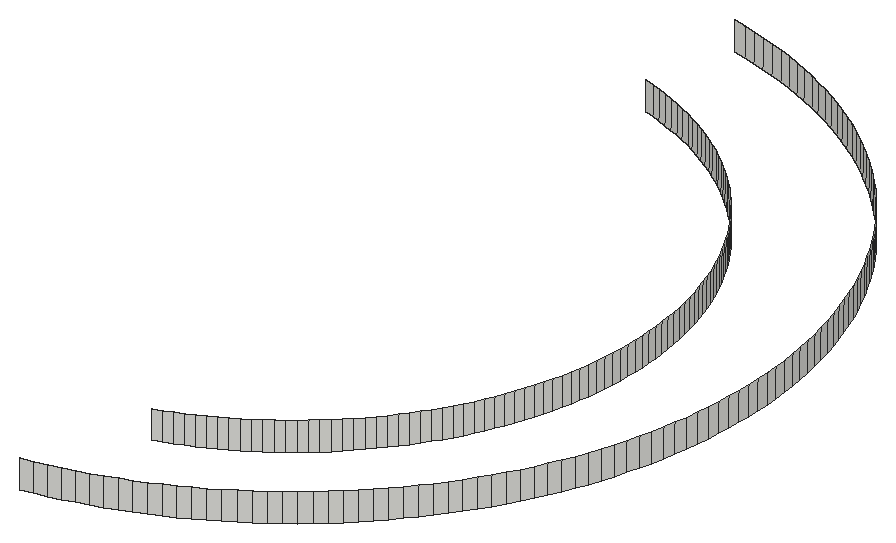
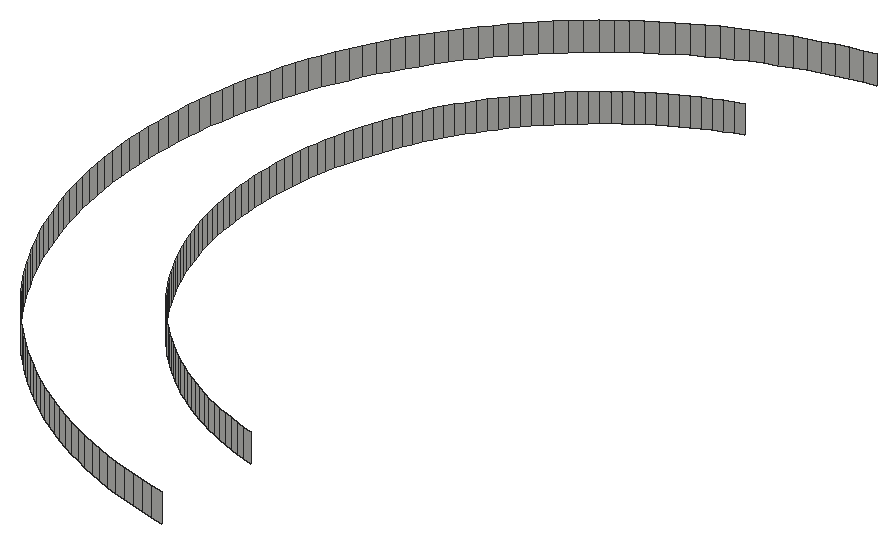
# SketchUp Ruby script. Lengths in inches.
U = 1.inch
M = Sketchup.active_model
def pt(a) = Geom::Point3d.new(a.map { |v| v * U })
def face(e, loops, mat)
  f = e.add_face(loops[0].map { |a| pt(a) })
  loops[1..].each { |l| e.add_face(l.map { |a| pt(a) }).erase! }
  f.material = f.back_material = mat if mat
  f
end
# faces: each face lists its corners as indices into pts; further lists are holes
def faces(e, pts, list, mat = nil) = list.each { |f| face(e, (f[0].is_a?(Array) ? f : [f]).map { |l| l.map { |i| pts[i] } }, mat) }
# xy, xz, yz: faces in a plane at the given z, y or x. An outline is a flat list of corners, or four numbers for a rectangle; further outlines are holes
def ring(l) = l.size == 4 ? [[l[0], l[1]], [l[2], l[1]], [l[2], l[3]], [l[0], l[3]]] : l.each_slice(2).to_a
def flat(e, list, mat, &to3) = list.each { |f| face(e, (f[0].is_a?(Array) ? f : [f]).map { |l| ring(l).map { |u, v| to3.(u, v) } }, mat) }
def xy(e, z, list, mat = nil) = flat(e, list, mat) { |x, y| [x, y, z] }
def xz(e, y, list, mat = nil) = flat(e, list, mat) { |x, z| [x, y, z] }
def yz(e, x, list, mat = nil) = flat(e, list, mat) { |y, z| [x, y, z] }
def lines(e, pts, list) = list.each { |a, b| e.add_line(pt(pts[a]), pt(pts[b])) }
# prism: a flat outline (further loops are holes) pulled along v
def prism(e, loops, v, mat = nil)
  f = face(e, loops, mat); d = Geom::Vector3d.new(v.map { |x| x * U })
  f.pushpull(f.normal.samedirection?(d) ? d.length : -d.length)
end
def box(e, o, s, mat = nil) = prism(e, [[o, [o[0] + s[0], o[1], o[2]], [o[0] + s[0], o[1] + s[1], o[2]], [o[0], o[1] + s[1], o[2]]]], [0, 0, s[2]], mat)
def at(x, y, z, deg = 0) = Geom::Transformation.translation(pt([x, y, z])) * Geom::Transformation.rotation(ORIGIN, Z_AXIS, deg.degrees)
def axes(o, x, y, z) = Geom::Transformation.new([*x, 0, *y, 0, *z, 0, *pt(o).to_a, 1])
def part(name) = M.definitions.add(name)
# library, detail: a bought-in or finely detailed component or shape, given as its bounding box
def library(name, o, s) = part(name).tap { |d| box(d.entities, o, s) }
def detail(e, o, s) = box(e.add_group.entities, o, s)
def put(e, d, t, mat = nil) = e.add_instance(d, t).tap { |i| i.material = mat if mat }
def group(e, t, mat = nil) = e.add_group.tap { |g| g.transformation = t; g.material = mat if mat }.entities
root = M.entities
p = [[923.47,230.86,117.3125],[925.9375,231.35,117.3125],[925.9375,231.35,111.3125],[923.47,230.86,111.3125],[928.39,231.91,117.3125],[928.39,231.91,111.3125],
  [930.83,232.53,117.3125],[930.83,232.53,111.3125],[933.24,233.21,117.3125],[933.24,233.21,111.3125],[935.64,233.95,117.3125],[935.64,233.95,111.3125],
  [938.02,234.76,117.3125],[938.02,234.76,111.3125],[940.38,235.63,117.3125],[940.38,235.63,111.3125],[942.72,236.5625,117.3125],[942.72,236.5625,111.3125],
  [945.03,237.56,117.3125],[945.03,237.56,111.3125],[947.31,238.61,117.3125],[947.31,238.61,111.3125],[949.5625,239.72,117.3125],[949.5625,239.72,111.3125],
  [951.79,240.89,117.3125],[951.79,240.89,111.3125],[953.98,242.12,117.3125],[953.98,242.12,111.3125],[956.14,243.4,117.3125],[956.14,243.4,111.3125],
  [958.26,244.74,117.3125],[958.26,244.74,111.3125],[960.35,246.14,117.3125],[960.35,246.14,111.3125],[962.41,247.59,117.3125],[962.41,247.59,111.3125],
  [964.42,249.09,117.3125],[964.42,249.09,111.3125],[966.39,250.65,117.3125],[966.39,250.65,111.3125],[968.33,252.26,117.3125],[968.33,252.26,111.3125],
  [970.22,253.91,117.3125],[970.22,253.91,111.3125],[972.0625,255.62,117.3125],[972.0625,255.62,111.3125],[973.86,257.375,117.3125],[973.86,257.375,111.3125],
  [931.78,258.04,117.3125],[930.01,257.39,117.3125],[930.01,257.39,111.3125],[931.78,258.04,111.3125],[975.61,259.17,117.3125],[975.61,259.17,111.3125],
  [933.53,258.74,117.3125],[933.53,258.74,111.3125],[935.26,259.48,117.3125],[935.26,259.48,111.3125],[977.32,261.02,117.3125],[977.32,261.02,111.3125],
  [936.98,260.27,117.3125],[936.98,260.27,111.3125],[938.67,261.1,117.3125],[938.67,261.1,111.3125],[978.98,262.91,117.3125],[978.98,262.91,111.3125],
  [940.33,261.98,117.3125],[940.33,261.98,111.3125],[941.98,262.9,117.3125],[941.98,262.9,111.3125],[943.6,263.87,117.3125],[943.6,263.87,111.3125],
  [980.58,264.84,117.3125],[980.58,264.84,111.3125],[945.19,264.87,117.3125],[945.19,264.87,111.3125],[982.14,266.82,117.3125],[982.14,266.82,111.3125],
  [946.76,265.92,117.3125],[946.76,265.92,111.3125],[948.3,267.01,117.3125],[948.3,267.01,111.3125],[983.64,268.83,117.3125],[983.64,268.83,111.3125],
  [949.81,268.13,117.3125],[949.81,268.13,111.3125],[951.29,269.3,117.3125],[951.29,269.3,111.3125],[985.09,270.88,117.3125],[985.09,270.88,111.3125],
  [952.74,270.51,117.3125],[952.74,270.51,111.3125],[954.16,271.75,117.3125],[954.16,271.75,111.3125],[986.49,272.97,117.3125],[986.49,272.97,111.3125],
  [955.54,273.03,117.3125],[955.54,273.03,111.3125],[956.89,274.34,117.3125],[956.89,274.34,111.3125],[987.83,275.1,117.3125],[987.83,275.1,111.3125],
  [958.21,275.69,117.3125],[958.21,275.69,111.3125],[989.12,277.26,117.3125],[989.12,277.26,111.3125],[959.49,277.08,117.3125],[959.49,277.08,111.3125],
  [960.73,278.5,117.3125],[960.73,278.5,111.3125],[990.35,279.45,117.3125],[990.35,279.45,111.3125],[961.93,279.95,117.3125],[961.93,279.95,111.3125],
  [991.52,281.67,117.3125],[991.52,281.67,111.3125],[963.1,281.43,117.3125],[963.1,281.43,111.3125],[964.23,282.9375,117.3125],[964.23,282.9375,111.3125],
  [992.625,283.93,117.3125],[992.625,283.93,111.3125],[965.32,284.47,117.3125],[965.32,284.47,111.3125],[993.68,286.21,117.3125],[993.68,286.21,111.3125],
  [966.36,286.04,117.3125],[966.36,286.04,111.3125],[967.37,287.64,117.3125],[967.37,287.64,111.3125],[994.67,288.52,117.3125],[994.67,288.52,111.3125],
  [968.33,289.26,117.3125],[968.33,289.26,111.3125],[995.6,290.85,117.3125],[995.6,290.85,111.3125],[969.25,290.9,117.3125],[969.25,290.9,111.3125],
  [970.13,292.57,117.3125],[970.13,292.57,111.3125],[996.47,293.21,117.3125],[996.47,293.21,111.3125],[970.96,294.26,117.3125],[970.96,294.26,111.3125],
  [997.28,295.59,117.3125],[997.28,295.59,111.3125],[971.75,295.97,117.3125],[971.75,295.97,111.3125],[998.03,297.99,117.3125],[998.03,297.99,111.3125],
  [972.5,297.7,117.3125],[972.5,297.7,111.3125],[973.2,299.45,117.3125],[973.2,299.45,111.3125],[998.71,300.41,117.3125],[998.71,300.41,111.3125],
  [973.85,301.22,117.3125],[973.85,301.22,111.3125],[999.33,302.85,117.3125],[999.33,302.85,111.3125],[974.45,303.01,117.3125],[974.45,303.01,111.3125],
  [999.88,305.3,117.3125],[999.88,305.3,111.3125],[975.01,304.81,117.3125],[975.01,304.81,111.3125],[975.53,306.62,117.3125],[975.53,306.62,111.3125],
  [1000.37,307.76,117.3125],[1000.37,307.76,111.3125],[975.99,308.45,117.3125],[975.99,308.45,111.3125],[1000.8,310.24,117.3125],[1000.8,310.24,111.3125],
  [976.41,310.29,117.3125],[976.41,310.29,111.3125],[1001.16,312.73,117.3125],[1001.16,312.73,111.3125],[976.77,312.14,117.3125],[976.77,312.14,111.3125],
  [977.09,313.99,117.3125],[977.09,313.99,111.3125],[1001.45,315.22,117.3125],[1001.45,315.22,111.3125],[977.36,315.86,117.3125],[977.36,315.86,111.3125],
  [1001.68,317.72,117.3125],[1001.68,317.72,111.3125],[977.58,317.73,117.3125],[977.58,317.73,111.3125],[977.76,319.61,117.3125],[977.76,319.61,111.3125],
  [1001.85,320.23,117.3125],[1001.85,320.23,111.3125],[977.88,321.49,117.3125],[977.88,321.49,111.3125],[1001.95,322.74,117.3125],[1001.95,322.74,111.3125],
  [977.95,323.37,117.3125],[977.95,323.37,111.3125],[1001.98,325.26,117.3125],[1001.98,325.26,111.3125],[977.98,325.26,117.3125],[977.98,325.26,111.3125],
  [977.95,327.14,117.3125],[977.95,327.14,111.3125],[1001.95,327.77,117.3125],[1001.95,327.77,111.3125],[977.88,329.02,117.3125],[977.88,329.02,111.3125],
  [1001.85,330.28,117.3125],[1001.85,330.28,111.3125],[977.76,330.91,117.3125],[977.76,330.91,111.3125],[1001.68,332.79,117.3125],[1001.68,332.79,111.3125],
  [977.58,332.78,117.3125],[977.58,332.78,111.3125],[977.36,334.65,117.3125],[977.36,334.65,111.3125],[1001.45,335.29,117.3125],[1001.45,335.29,111.3125],
  [977.09,336.52,117.3125],[977.09,336.52,111.3125],[1001.16,337.79,117.3125],[1001.16,337.79,111.3125],[976.77,338.38,117.3125],[976.77,338.38,111.3125],
  [1000.8,340.27,117.3125],[1000.8,340.27,111.3125],[976.41,340.23,117.3125],[976.41,340.23,111.3125],[975.99,342.0625,117.3125],[975.99,342.0625,111.3125],
  [1000.37,342.75,117.3125],[1000.37,342.75,111.3125],[975.53,343.89,117.3125],[975.53,343.89,111.3125],[999.88,345.22,117.3125],[999.88,345.22,111.3125],
  [975.01,345.71,117.3125],[975.01,345.71,111.3125],[999.33,347.67,117.3125],[999.33,347.67,111.3125],[974.45,347.51,117.3125],[974.45,347.51,111.3125],
  [973.85,349.29,117.3125],[973.85,349.29,111.3125],[998.71,350.1,117.3125],[998.71,350.1,111.3125],[973.2,351.06,117.3125],[973.2,351.06,111.3125],
  [998.03,352.52,117.3125],[998.03,352.52,111.3125],[972.5,352.81,117.3125],[972.5,352.81,111.3125],[997.28,354.92,117.3125],[997.28,354.92,111.3125],
  [971.75,354.54,117.3125],[971.75,354.54,111.3125],[970.96,356.25,117.3125],[970.96,356.25,111.3125],[996.47,357.3,117.3125],[996.47,357.3,111.3125],
  [970.13,357.94,117.3125],[970.13,357.94,111.3125],[995.6,359.66,117.3125],[995.6,359.66,111.3125],[969.25,359.61,117.3125],[969.25,359.61,111.3125],
  [968.33,361.26,117.3125],[968.33,361.26,111.3125],[994.67,361.99,117.3125],[994.67,361.99,111.3125],[967.37,362.875,117.3125],[967.37,362.875,111.3125],
  [993.68,364.3,117.3125],[993.68,364.3,111.3125],[966.36,364.47,117.3125],[966.36,364.47,111.3125],[992.625,366.59,117.3125],[992.625,366.59,111.3125],
  [965.32,366.04,117.3125],[965.32,366.04,111.3125],[964.23,367.58,117.3125],[964.23,367.58,111.3125],[991.52,368.84,117.3125],[991.52,368.84,111.3125],
  [963.1,369.09,117.3125],[963.1,369.09,111.3125],[990.35,371.0625,117.3125],[990.35,371.0625,111.3125],[961.93,370.57,117.3125],[961.93,370.57,111.3125],
  [960.73,372.02,117.3125],[960.73,372.02,111.3125],[989.12,373.26,117.3125],[989.12,373.26,111.3125],[959.49,373.43,117.3125],[959.49,373.43,111.3125],
  [987.83,375.42,117.3125],[987.83,375.42,111.3125],[958.21,374.82,117.3125],[958.21,374.82,111.3125],[956.89,376.17,117.3125],[956.89,376.17,111.3125],
  [986.49,377.54,117.3125],[986.49,377.54,111.3125],[955.54,377.48,117.3125],[955.54,377.48,111.3125],[954.16,378.76,117.3125],[954.16,378.76,111.3125],
  [985.09,379.63,117.3125],[985.09,379.63,111.3125],[952.74,380.01,117.3125],[952.74,380.01,111.3125],[983.64,381.68,117.3125],[983.64,381.68,111.3125],
  [951.29,381.21,117.3125],[951.29,381.21,111.3125],[949.81,382.38,117.3125],[949.81,382.38,111.3125],[982.14,383.7,117.3125],[982.14,383.7,111.3125],
  [948.3,383.51,117.3125],[948.3,383.51,111.3125],[946.76,384.59,117.3125],[946.76,384.59,111.3125],[980.58,385.67,117.3125],[980.58,385.67,111.3125],
  [945.19,385.64,117.3125],[945.19,385.64,111.3125],[943.6,386.65,117.3125],[943.6,386.65,111.3125],[978.98,387.6,117.3125],[978.98,387.6,111.3125],
  [941.98,387.61,117.3125],[941.98,387.61,111.3125],[940.33,388.53,117.3125],[940.33,388.53,111.3125],[977.32,389.49,117.3125],[977.32,389.49,111.3125],
  [938.67,389.41,117.3125],[938.67,389.41,111.3125],[936.98,390.24,117.3125],[936.98,390.24,111.3125],[975.61,391.34,117.3125],[975.61,391.34,111.3125],
  [935.26,391.03,117.3125],[935.26,391.03,111.3125],[933.53,391.78,117.3125],[933.53,391.78,111.3125],[973.86,393.14,117.3125],[973.86,393.14,111.3125],
  [931.78,392.47,117.3125],[931.78,392.47,111.3125],[930.01,393.125,117.3125],[930.01,393.125,111.3125],[928.23,393.73,117.3125],[928.23,393.73,111.3125],
  [972.0625,394.89,117.3125],[972.0625,394.89,111.3125],[926.43,394.29,117.3125],[926.43,394.29,111.3125],[924.61,394.8,117.3125],[924.61,394.8,111.3125],
  [970.22,396.6,117.3125],[970.22,396.6,111.3125],[968.33,398.26,117.3125],[968.33,398.26,111.3125],[966.39,399.86,117.3125],[966.39,399.86,111.3125],
  [964.42,401.42,117.3125],[964.42,401.42,111.3125],[962.41,402.92,117.3125],[962.41,402.92,111.3125],[960.35,404.37,117.3125],[960.35,404.37,111.3125],
  [958.26,405.77,117.3125],[958.26,405.77,111.3125],[956.14,407.11,117.3125],[956.14,407.11,111.3125],[953.98,408.39,117.3125],[953.98,408.39,111.3125],
  [951.79,409.62,117.3125],[951.79,409.62,111.3125],[949.5625,410.79,117.3125],[949.5625,410.79,111.3125],[947.31,411.9,117.3125],[947.31,411.9,111.3125],
  [945.03,412.96,117.3125],[945.03,412.96,111.3125],[942.72,413.95,117.3125],[942.72,413.95,111.3125],[940.38,414.88,117.3125],[940.38,414.88,111.3125],
  [938.02,415.75,117.3125],[938.02,415.75,111.3125],[935.64,416.56,117.3125],[935.64,416.56,111.3125],[933.24,417.3,117.3125],[933.24,417.3,111.3125],
  [930.83,417.99,117.3125],[930.83,417.99,111.3125],[928.39,418.6,117.3125],[928.39,418.6,111.3125],[925.9375,419.16,117.3125],[925.9375,419.16,111.3125],
  [923.47,419.65,117.3125],[923.47,419.65,111.3125]]
faces(root,p,[[0,1,2,3],[1,4,5,2],[4,6,7,5],[6,8,9,7],[8,10,11,9],[10,12,13,11],[12,14,15,13],[14,16,17,15],
  [16,18,19,17],[18,20,21,19],[20,22,23,21],[22,24,25,23],[24,26,27,25],[26,28,29,27],[28,30,31,29],[30,32,33,31],
  [32,34,35,33],[34,36,37,35],[36,38,39,37],[38,40,41,39],[40,42,43,41],[42,44,45,43],[44,46,47,45],[48,49,50,51],
  [46,52,53,47],[54,48,51,55],[56,54,55,57],[52,58,59,53],[60,56,57,61],[62,60,61,63],[58,64,65,59],[66,62,63,67],
  [68,66,67,69],[70,68,69,71],[64,72,73,65],[74,70,71,75],[72,76,77,73],[78,74,75,79],[80,78,79,81],[76,82,83,77],
  [84,80,81,85],[86,84,85,87],[82,88,89,83],[90,86,87,91],[92,90,91,93],[88,94,95,89],[96,92,93,97],[98,96,97,99],
  [94,100,101,95],[102,98,99,103],[100,104,105,101],[106,102,103,107],[108,106,107,109],[104,110,111,105],[112,108,109,113],[110,114,115,111],
  [116,112,113,117],[118,116,117,119],[114,120,121,115],[122,118,119,123],[120,124,125,121],[126,122,123,127],[128,126,127,129],[124,130,131,125],
  [132,128,129,133],[130,134,135,131],[136,132,133,137],[138,136,137,139],[134,140,141,135],[142,138,139,143],[140,144,145,141],[146,142,143,147],
  [144,148,149,145],[150,146,147,151],[152,150,151,153],[148,154,155,149],[156,152,153,157],[154,158,159,155],[160,156,157,161],[158,162,163,159],
  [164,160,161,165],[166,164,165,167],[162,168,169,163],[170,166,167,171],[168,172,173,169],[174,170,171,175],[172,176,177,173],[178,174,175,179],
  [180,178,179,181],[176,182,183,177],[184,180,181,185],[182,186,187,183],[188,184,185,189],[190,188,189,191],[186,192,193,187],[194,190,191,195],
  [192,196,197,193],[198,194,195,199],[196,200,201,197],[202,198,199,203],[204,202,203,205],[200,206,207,201],[208,204,205,209],[206,210,211,207],
  [212,208,209,213],[210,214,215,211],[216,212,213,217],[218,216,217,219],[214,220,221,215],[222,218,219,223],[220,224,225,221],[226,222,223,227],
  [224,228,229,225],[230,226,227,231],[232,230,231,233],[228,234,235,229],[236,232,233,237],[234,238,239,235],[240,236,237,241],[238,242,243,239],
  [244,240,241,245],[246,244,245,247],[242,248,249,243],[250,246,247,251],[248,252,253,249],[254,250,251,255],[252,256,257,253],[258,254,255,259],
  [260,258,259,261],[256,262,263,257],[264,260,261,265],[262,266,267,263],[268,264,265,269],[270,268,269,271],[266,272,273,267],[274,270,271,275],
  [272,276,277,273],[278,274,275,279],[276,280,281,277],[282,278,279,283],[284,282,283,285],[280,286,287,281],[288,284,285,289],[286,290,291,287],
  [292,288,289,293],[294,292,293,295],[290,296,297,291],[298,294,295,299],[296,300,301,297],[302,298,299,303],[304,302,303,305],[300,306,307,301],
  [308,304,305,309],[310,308,309,311],[306,312,313,307],[314,310,311,315],[312,316,317,313],[318,314,315,319],[320,318,319,321],[316,322,323,317],
  [324,320,321,325],[326,324,325,327],[322,328,329,323],[330,326,327,331],[332,330,331,333],[328,334,335,329],[336,332,333,337],[338,336,337,339],
  [334,340,341,335],[342,338,339,343],[344,342,343,345],[340,346,347,341],[348,344,345,349],[350,348,349,351],[346,352,353,347],[354,350,351,355],
  [356,354,355,357],[358,356,357,359],[352,360,361,353],[362,358,359,363],[364,362,363,365],[360,366,367,361],[366,368,369,367],[368,370,371,369],
  [370,372,373,371],[372,374,375,373],[374,376,377,375],[376,378,379,377],[378,380,381,379],[380,382,383,381],[382,384,385,383],[384,386,387,385],
  [386,388,389,387],[388,390,391,389],[390,392,393,391],[392,394,395,393],[394,396,397,395],[396,398,399,397],[398,400,401,399],[400,402,403,401],
  [402,404,405,403],[404,406,407,405],[406,408,409,407]])
